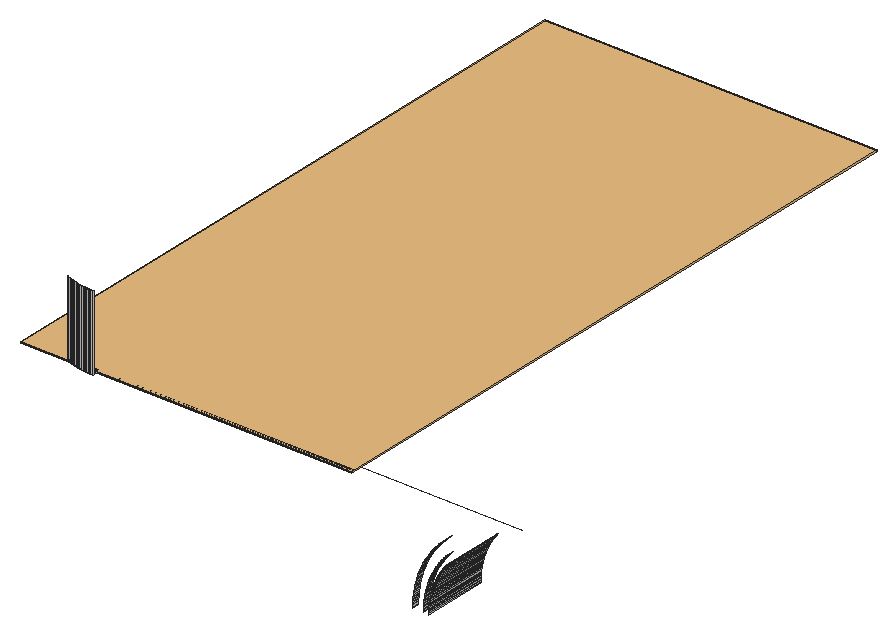
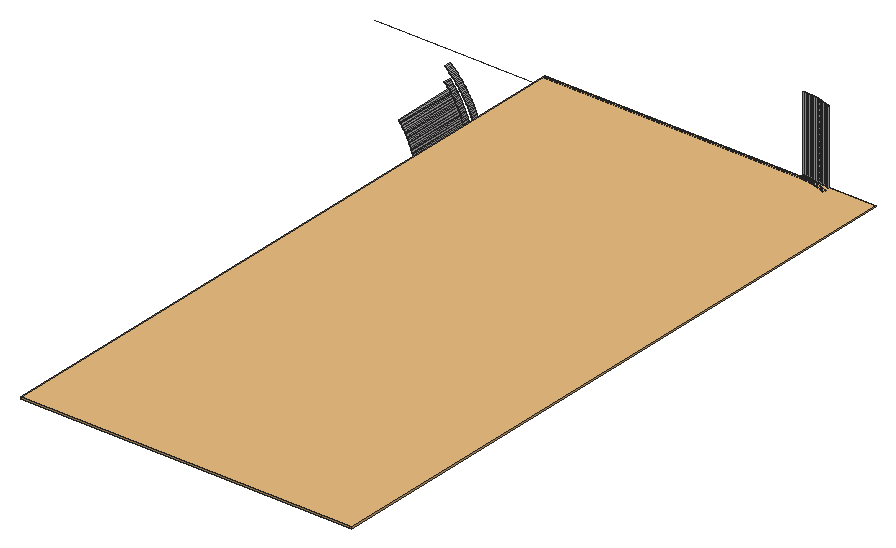
# SketchUp Ruby script. Lengths in inches.
U = 1.inch
M = Sketchup.active_model
def pt(a) = Geom::Point3d.new(a.map { |v| v * U })
def face(e, loops, mat)
  f = e.add_face(loops[0].map { |a| pt(a) })
  loops[1..].each { |l| e.add_face(l.map { |a| pt(a) }).erase! }
  f.material = f.back_material = mat if mat
  f
end
# faces: each face lists its corners as indices into pts; further lists are holes
def faces(e, pts, list, mat = nil) = list.each { |f| face(e, (f[0].is_a?(Array) ? f : [f]).map { |l| l.map { |i| pts[i] } }, mat) }
# xy, xz, yz: faces in a plane at the given z, y or x. An outline is a flat list of corners, or four numbers for a rectangle; further outlines are holes
def ring(l) = l.size == 4 ? [[l[0], l[1]], [l[2], l[1]], [l[2], l[3]], [l[0], l[3]]] : l.each_slice(2).to_a
def flat(e, list, mat, &to3) = list.each { |f| face(e, (f[0].is_a?(Array) ? f : [f]).map { |l| ring(l).map { |u, v| to3.(u, v) } }, mat) }
def xy(e, z, list, mat = nil) = flat(e, list, mat) { |x, y| [x, y, z] }
def xz(e, y, list, mat = nil) = flat(e, list, mat) { |x, z| [x, y, z] }
def yz(e, x, list, mat = nil) = flat(e, list, mat) { |y, z| [x, y, z] }
def lines(e, pts, list) = list.each { |a, b| e.add_line(pt(pts[a]), pt(pts[b])) }
# prism: a flat outline (further loops are holes) pulled along v
def prism(e, loops, v, mat = nil)
  f = face(e, loops, mat); d = Geom::Vector3d.new(v.map { |x| x * U })
  f.pushpull(f.normal.samedirection?(d) ? d.length : -d.length)
end
def box(e, o, s, mat = nil) = prism(e, [[o, [o[0] + s[0], o[1], o[2]], [o[0] + s[0], o[1] + s[1], o[2]], [o[0], o[1] + s[1], o[2]]]], [0, 0, s[2]], mat)
def at(x, y, z, deg = 0) = Geom::Transformation.translation(pt([x, y, z])) * Geom::Transformation.rotation(ORIGIN, Z_AXIS, deg.degrees)
def axes(o, x, y, z) = Geom::Transformation.new([*x, 0, *y, 0, *z, 0, *pt(o).to_a, 1])
def part(name) = M.definitions.add(name)
# library, detail: a bought-in or finely detailed component or shape, given as its bounding box
def library(name, o, s) = part(name).tap { |d| box(d.entities, o, s) }
def detail(e, o, s) = box(e.add_group.entities, o, s)
def put(e, d, t, mat = nil) = e.add_instance(d, t).tap { |i| i.material = mat if mat }
def group(e, t, mat = nil) = e.add_group.tap { |g| g.transformation = t; g.material = mat if mat }.entities
root = M.entities
M.materials.add("Outer Light - 1").color = [251, 216, 141]
M.materials.add("[Quartz Light Brown]").color = [215, 212, 212]
c1 = library("Group\#10",[0,0,0],[61.75,122.25,0.25])
xz(root,143,[[215.8,354,216,368]],"[Quartz Light Brown]")
xz(root,143.01,[[215.41,354,215.61,368]],"[Quartz Light Brown]")
xz(root,143.75,[[215.625,354,215.8125,354.25],[215.8125,354,216,354.25],[216,354,263.5,354.25]],"[Quartz Light Brown]")
xz(root,144.25,[[215.64,354,215.82,354.25],[215.82,354,216,354.25],[216,354,263.5,354.25]],"[Quartz Light Brown]")
yz(root,275.5,[[143,336,144.25,336.24]],"[Quartz Light Brown]")
yz(root,275.51,[[143,336.47,144.25,336.71]],"[Quartz Light Brown]")
yz(root,277.5,[[143,336,144.25,336.21]],"[Quartz Light Brown]")
yz(root,277.51,[[143,336.42,144.25,336.63]],"[Quartz Light Brown]")
yz(root,278.5,[[143,336,155,336.2]],"[Quartz Light Brown]")
yz(root,278.51,[[143,336.39,155,336.59]],"[Quartz Light Brown]")
p = [[275.51,144.25,336.47],[275.51,143,336.47],[275.5,143,336.24],[275.5,144.25,336.24],[277.5,143,336.21],[277.51,143,336.42],
  [277.51,144.25,336.42],[277.5,144.25,336.21],[278.51,143,336.39],[278.5,143,336.2],[278.5,155,336.2],[278.51,155,336.39],
  [277.51,143,336.63],[277.52,143,336.84],[277.52,144.25,336.84],[277.51,144.25,336.63],[278.52,143,336.79],[278.51,143,336.59],
  [278.51,155,336.59],[278.52,155,336.79],[275.52,144.25,336.94],[275.52,143,336.94],[275.51,143,336.71],[275.51,144.25,336.71],
  [277.53,143,337.05],[277.53,144.25,337.05],[278.53,143,336.98],[278.53,155,336.98],[275.54,144.25,337.18],[275.54,143,337.18],
  [277.55,143,337.26],[277.55,144.25,337.26],[278.55,143,337.18],[278.55,155,337.18],[275.56,144.25,337.41],[275.56,143,337.41],
  [278.5625,143,337.37],[278.5625,155,337.37],[277.57,143,337.46],[277.57,144.25,337.46],[275.58,144.25,337.65],[275.58,143,337.65],
  [278.58,143,337.57],[278.58,155,337.57],[277.59,143,337.67],[277.59,144.25,337.67],[275.6,144.25,337.88],[275.6,143,337.88],
  [278.6,143,337.76],[278.6,155,337.76],[277.61,143,337.88],[277.61,144.25,337.88],[278.63,143,337.96],[278.63,155,337.96],
  [275.625,144.25,338.12],[275.625,143,338.12],[277.64,143,338.09],[277.64,144.25,338.09],[278.66,143,338.15],[278.66,155,338.15],
  [275.65,144.25,338.35],[275.65,143,338.35],[277.67,143,338.3],[277.67,144.25,338.3],[278.68,143,338.35],[278.68,155,338.35],
  [275.6875,144.25,338.58],[275.6875,143,338.58],[277.7,143,338.5],[277.7,144.25,338.5],[278.72,143,338.54],[278.72,155,338.54],
  [277.73,143,338.71],[277.73,144.25,338.71],[278.75,143,338.73],[278.75,155,338.73],[275.72,144.25,338.82],[275.72,143,338.82],
  [277.77,143,338.92],[277.77,144.25,338.92],[278.79,143,338.93],[278.79,155,338.93],[275.76,144.25,339.05],[275.76,143,339.05],
  [277.81,143,339.12],[277.81,144.25,339.12],[278.83,143,339.12],[278.83,155,339.12],[275.8,144.25,339.28],[275.8,143,339.28],
  [277.85,143,339.33],[277.85,144.25,339.33],[278.87,143,339.31],[278.87,155,339.31],[275.85,144.25,339.51],[275.85,143,339.51],
  [277.89,143,339.53],[277.89,144.25,339.53],[278.91,143,339.5],[278.91,155,339.5],[275.89,144.25,339.74],[275.89,143,339.74],
  [277.94,143,339.74],[277.94,144.25,339.74],[278.96,143,339.69],[278.96,155,339.69],[275.94,144.25,339.97],[275.94,143,339.97],
  [277.99,143,339.9375],[277.99,144.25,339.9375],[279.01,143,339.88],[279.01,155,339.88],[278.05,143,340.14],[278.05,144.25,340.14],
  [279.0625,143,340.07],[279.0625,155,340.07],[276,144.25,340.2],[276,143,340.2],[278.1,143,340.34],[278.1,144.25,340.34],
  [279.12,143,340.26],[279.12,155,340.26],[276.05,144.25,340.43],[276.05,143,340.43],[278.16,143,340.54],[278.16,144.25,340.54],
  [279.17,143,340.45],[279.17,155,340.45],[276.11,144.25,340.66],[276.11,143,340.66],[279.23,143,340.64],[279.23,155,340.64],
  [278.22,143,340.74],[278.22,144.25,340.74],[279.3,143,340.82],[279.3,155,340.82],[276.18,144.25,340.89],[276.18,143,340.89],
  [278.28,143,340.94],[278.28,144.25,340.94],[279.36,143,341.01],[279.36,155,341.01],[276.24,144.25,341.11],[276.24,143,341.11],
  [278.35,143,341.14],[278.35,144.25,341.14],[279.43,143,341.19],[279.43,155,341.19],[276.31,144.25,341.34],[276.31,143,341.34],
  [278.42,143,341.34],[278.42,144.25,341.34],[279.5,143,341.375],[279.5,155,341.375],[276.38,144.25,341.5625],[276.38,143,341.5625],
  [278.49,143,341.54],[278.49,144.25,341.54],[279.57,143,341.56],[279.57,155,341.56],[278.5625,143,341.73],[278.5625,144.25,341.73],
  [276.46,144.25,341.79],[276.46,143,341.79],[279.64,143,341.74],[279.64,155,341.74],[278.64,143,341.93],[278.64,144.25,341.93],
  [279.72,143,341.92],[279.72,155,341.92],[276.53,144.25,342.01],[276.53,143,342.01],[278.72,143,342.12],[278.72,144.25,342.12],
  [279.8,143,342.1],[279.8,155,342.1],[276.61,144.25,342.23],[276.61,143,342.23],[278.8,143,342.32],[278.8,144.25,342.32],
  [279.88,143,342.28],[279.88,155,342.28],[276.7,144.25,342.45],[276.7,143,342.45],[278.88,143,342.51],[278.88,144.25,342.51],
  [279.96,143,342.46],[279.96,155,342.46],[276.78,144.25,342.67],[276.78,143,342.67],[278.97,143,342.7],[278.97,144.25,342.7],
  [280.05,143,342.63],[280.05,155,342.63],[280.13,143,342.81],[280.13,155,342.81],[276.87,144.25,342.89],[276.87,143,342.89],
  [279.06,143,342.89],[279.06,144.25,342.89],[280.23,143,342.98],[280.23,155,342.98],[276.96,144.25,343.11],[276.96,143,343.11],
  [279.15,143,343.08],[279.15,144.25,343.08],[280.32,143,343.16],[280.32,155,343.16],[277.06,144.25,343.32],[277.06,143,343.32],
  [279.24,143,343.26],[279.24,144.25,343.26],[280.41,143,343.33],[280.41,155,343.33],[277.15,144.25,343.54],[277.15,143,343.54],
  [279.34,143,343.45],[279.34,144.25,343.45],[280.51,143,343.5],[280.51,155,343.5],[279.4375,143,343.63],[279.4375,144.25,343.63],
  [277.25,144.25,343.75],[277.25,143,343.75],[280.61,143,343.67],[280.61,155,343.67],[279.54,143,343.82],[279.54,144.25,343.82],
  [277.36,144.25,343.96],[277.36,143,343.96],[280.71,143,343.84],[280.71,155,343.84],[279.64,143,344],[279.64,144.25,344],
  [280.8125,143,344],[280.8125,155,344],[277.46,144.25,344.17],[277.46,143,344.17],[279.75,143,344.18],[279.75,144.25,344.18],
  [280.92,143,344.17],[280.92,155,344.17],[277.57,144.25,344.38],[277.57,143,344.38],[279.86,143,344.36],[279.86,144.25,344.36],
  [281.03,143,344.33],[281.03,155,344.33],[281.14,143,344.5],[281.14,155,344.5],[277.68,144.25,344.59],[277.68,143,344.59],
  [279.97,143,344.54],[279.97,144.25,344.54],[280.08,143,344.71],[280.08,144.25,344.71],[281.25,143,344.66],[281.25,155,344.66],
  [277.8,144.25,344.8],[277.8,143,344.8],[280.2,143,344.89],[280.2,144.25,344.89],[281.36,143,344.82],[281.36,155,344.82],
  [277.91,144.25,345],[277.91,143,345],[281.48,143,344.97],[281.48,155,344.97],[280.3125,143,345.0625],[280.3125,144.25,345.0625],
  [278.03,144.25,345.2],[278.03,143,345.2],[281.6,143,345.13],[281.6,155,345.13],[280.43,143,345.23],[280.43,144.25,345.23],
  [281.72,143,345.29],[281.72,155,345.29],[278.15,144.25,345.4],[278.15,143,345.4],[280.56,143,345.4],[280.56,144.25,345.4],
  [281.84,143,345.44],[281.84,155,345.44],[278.28,144.25,345.61],[278.28,143,345.61],[280.68,143,345.57],[280.68,144.25,345.57],
  [278.4,144.25,345.8],[278.4,143,345.8],[280.81,143,345.74],[280.81,144.25,345.74],[280.93,143,345.91],[280.93,144.25,345.91],
  [278.53,144.25,346],[278.53,143,346],[281.07,143,346.07],[281.07,144.25,346.07],[278.67,144.25,346.2],[278.67,143,346.2],
  [281.2,143,346.23],[281.2,144.25,346.23],[278.8,144.25,346.39],[278.8,143,346.39],[281.33,143,346.39],[281.33,144.25,346.39],
  [278.9375,144.25,346.58],[278.9375,143,346.58],[281.47,143,346.55],[281.47,144.25,346.55],[281.61,143,346.71],[281.61,144.25,346.71],
  [279.08,144.25,346.77],[279.08,143,346.77],[281.75,143,346.86],[281.75,144.25,346.86],[279.22,144.25,346.96],[279.22,143,346.96],
  [281.89,143,347.01],[281.89,144.25,347.01],[279.36,144.25,347.14],[279.36,143,347.14],[279.51,144.25,347.33],[279.51,143,347.33],
  [279.66,144.25,347.51],[279.66,143,347.51],[279.8125,144.25,347.69],[279.8125,143,347.69],[279.97,144.25,347.87],[279.97,143,347.87],
  [280.125,144.25,348.04],[280.125,143,348.04],[280.28,144.25,348.22],[280.28,143,348.22],[280.44,144.25,348.39],[280.44,143,348.39],
  [280.61,144.25,348.56],[280.61,143,348.56],[280.77,144.25,348.73],[280.77,143,348.73],[280.94,144.25,348.89],[280.94,143,348.89],
  [281.11,144.25,349.06],[281.11,143,349.06],[281.28,144.25,349.22],[281.28,143,349.22],[281.46,144.25,349.375],[281.46,143,349.375],
  [281.63,144.25,349.53],[281.63,143,349.53],[281.81,144.25,349.6875],[281.81,143,349.6875],[214.63,143.0625,368],[214.63,143.0625,354],
  [214.82,143.05,354],[214.82,143.05,368],[215.02,143.03,354],[215.02,143.03,368],[215.21,143.02,354],[215.21,143.02,368],
  [215.41,143.01,354],[215.41,143.01,368],[215.61,143.01,368],[215.61,143.01,354],[215.8,143,354],[215.8,143,368],
  [213.85,143.16,368],[213.85,143.16,354],[214.04,143.13,354],[214.04,143.13,368],[214.24,143.1,354],[214.24,143.1,368],
  [214.43,143.08,354],[214.43,143.08,368],[213.27,143.25,368],[213.27,143.25,354],[213.46,143.22,354],[213.46,143.22,368],
  [213.65,143.18,354],[213.65,143.18,368],[212.69,143.37,368],[212.69,143.37,354],[212.88,143.33,354],[212.88,143.33,368],
  [213.07,143.29,354],[213.07,143.29,368],[212.31,143.46,368],[212.31,143.46,354],[212.5,143.41,354],[212.5,143.41,368],
  [211.93,143.5625,368],[211.93,143.5625,354],[212.12,143.51,354],[212.12,143.51,368],[211.55,143.67,368],[211.55,143.67,354],
  [211.74,143.62,354],[211.74,143.62,368],[211.18,143.8,368],[211.18,143.8,354],[211.36,143.73,354],[211.36,143.73,368],
  [210.99,143.86,368],[210.99,143.86,354],[214.33,143.85,354],[214.14,143.87,354],[214.14,143.87,354.25],[214.33,143.85,354.25],
  [214.51,143.83,354],[214.51,143.83,354.25],[214.7,143.81,354],[214.7,143.81,354.25],[214.88,143.79,354],[214.88,143.79,354.25],
  [215.07,143.78,354],[215.07,143.78,354.25],[215.25,143.77,354],[215.25,143.77,354.25],[215.44,143.76,354],[215.44,143.76,354.25],
  [215.625,143.75,354],[215.625,143.75,354.25],[210.625,144,368],[210.625,144,354],[210.81,143.93,354],[210.81,143.93,368],
  [213.77,143.93,354],[213.59,143.96,354],[213.59,143.96,354.25],[213.77,143.93,354.25],[213.96,143.9,354],[213.96,143.9,354.25],
  [210.44,144.07,368],[210.44,144.07,354],[213.22,144.02,354],[213.04,144.0625,354],[213.04,144.0625,354.25],[213.22,144.02,354.25],
  [213.4,143.99,354],[213.4,143.99,354.25],[210.26,144.14,368],[210.26,144.14,354],[212.67,144.14,354],[212.49,144.1875,354],
  [212.49,144.1875,354.25],[212.67,144.14,354.25],[212.86,144.1,354],[212.86,144.1,354.25],[212.3125,144.24,354],[212.13,144.29,354],
  [212.13,144.29,354.25],[212.3125,144.24,354.25],[211.95,144.34,354],[211.77,144.39,354],[211.77,144.39,354.25],[211.95,144.34,354.25],
  [214.21,144.37,354],[214.38,144.35,354],[214.38,144.35,354.25],[214.21,144.37,354.25],[214.5625,144.33,354],[214.5625,144.33,354.25],
  [214.74,144.31,354],[214.74,144.31,354.25],[214.92,144.29,354],[214.92,144.29,354.25],[215.1,144.28,354],[215.1,144.28,354.25],
  [215.28,144.27,354],[215.28,144.27,354.25],[215.46,144.26,354],[215.46,144.26,354.25],[215.64,144.25,354],[215.64,144.25,354.25],
  [211.6,144.45,354],[211.42,144.51,354],[211.42,144.51,354.25],[211.6,144.45,354.25],[213.49,144.48,354],[213.67,144.45,354],
  [213.67,144.45,354.25],[213.49,144.48,354.25],[213.85,144.42,354],[213.85,144.42,354.25],[214.03,144.39,354],[214.03,144.39,354.25],
  [211.24,144.57,354],[211.24,144.57,354.25],[213.14,144.55,354],[213.32,144.51,354],[213.32,144.51,354.25],[213.14,144.55,354.25],
  [211.07,144.63,354],[210.89,144.7,354],[210.89,144.7,354.25],[211.07,144.63,354.25],[212.62,144.67,354],[212.79,144.63,354],
  [212.79,144.63,354.25],[212.62,144.67,354.25],[212.97,144.59,354],[212.97,144.59,354.25],[210.72,144.76,354],[210.72,144.76,354.25],
  [212.27,144.77,354],[212.44,144.72,354],[212.44,144.72,354.25],[212.27,144.77,354.25],[210.55,144.83,354],[210.375,144.91,354],
  [210.375,144.91,354.25],[210.55,144.83,354.25],[211.92,144.87,354],[212.09,144.82,354],[212.09,144.82,354.25],[211.92,144.87,354.25],
  [210.2,144.98,354],[210.2,144.98,354.25],[211.58,144.98,354],[211.75,144.92,354],[211.75,144.92,354.25],[211.58,144.98,354.25],
  [211.24,145.1,354],[211.41,145.04,354],[211.41,145.04,354.25],[211.24,145.1,354.25],[211.07,145.16,354],[211.07,145.16,354.25],
  [210.74,145.3,354],[210.9,145.23,354],[210.9,145.23,354.25],[210.74,145.3,354.25],[210.57,145.37,354],[210.57,145.37,354.25],
  [210.24,145.51,354],[210.41,145.4375,354],[210.41,145.4375,354.25],[210.24,145.51,354.25],[263.5,146,354],[293.5,146,354]]
faces(root,p,[[0,1,2,3],[4,5,6,7],[8,9,10,11],[12,13,14,15],[16,17,18,19],[20,21,22,23],[13,24,25,14],[26,16,19,27],
  [28,29,21,20],[24,30,31,25],[32,26,27,33],[34,35,29,28],[36,32,33,37],[30,38,39,31],[40,41,35,34],[42,36,37,43],
  [38,44,45,39],[46,47,41,40],[48,42,43,49],[44,50,51,45],[52,48,49,53],[54,55,47,46],[50,56,57,51],[58,52,53,59],
  [60,61,55,54],[56,62,63,57],[64,58,59,65],[66,67,61,60],[62,68,69,63],[70,64,65,71],[68,72,73,69],[74,70,71,75],
  [76,77,67,66],[72,78,79,73],[80,74,75,81],[82,83,77,76],[78,84,85,79],[86,80,81,87],[88,89,83,82],[84,90,91,85],
  [92,86,87,93],[94,95,89,88],[90,96,97,91],[98,92,93,99],[100,101,95,94],[96,102,103,97],[104,98,99,105],[106,107,101,100],
  [102,108,109,103],[110,104,105,111],[108,112,113,109],[114,110,111,115],[116,117,107,106],[112,118,119,113],[120,114,115,121],[122,123,117,116],
  [118,124,125,119],[126,120,121,127],[128,129,123,122],[130,126,127,131],[124,132,133,125],[134,130,131,135],[136,137,129,128],[132,138,139,133],
  [140,134,135,141],[142,143,137,136],[138,144,145,139],[146,140,141,147],[148,149,143,142],[144,150,151,145],[152,146,147,153],[154,155,149,148],
  [150,156,157,151],[158,152,153,159],[156,160,161,157],[162,163,155,154],[164,158,159,165],[160,166,167,161],[168,164,165,169],[170,171,163,162],
  [166,172,173,167],[174,168,169,175],[176,177,171,170],[172,178,179,173],[180,174,175,181],[182,183,177,176],[178,184,185,179],[186,180,181,187],
  [188,189,183,182],[184,190,191,185],[192,186,187,193],[194,192,193,195],[196,197,189,188],[190,198,199,191],[200,194,195,201],[202,203,197,196],
  [198,204,205,199],[206,200,201,207],[208,209,203,202],[204,210,211,205],[212,206,207,213],[214,215,209,208],[210,216,217,211],[218,212,213,219],
  [216,220,221,217],[222,223,215,214],[224,218,219,225],[220,226,227,221],[228,229,223,222],[230,224,225,231],[226,232,233,227],[234,230,231,235],
  [236,237,229,228],[232,238,239,233],[240,234,235,241],[242,243,237,236],[238,244,245,239],[246,240,241,247],[248,246,247,249],[250,251,243,242],
  [244,252,253,245],[252,254,255,253],[256,248,249,257],[258,259,251,250],[254,260,261,255],[262,256,257,263],[264,265,259,258],[266,262,263,267],
  [260,268,269,261],[270,271,265,264],[272,266,267,273],[268,274,275,269],[276,272,273,277],[278,279,271,270],[274,280,281,275],[282,276,277,283],
  [284,285,279,278],[280,286,287,281],[288,289,285,284],[286,290,291,287],[290,292,293,291],[294,295,289,288],[292,296,297,293],[298,299,295,294],
  [296,300,301,297],[302,303,299,298],[300,304,305,301],[306,307,303,302],[304,308,309,305],[308,310,311,309],[312,313,307,306],[310,314,315,311],
  [316,317,313,312],[314,318,319,315],[320,321,317,316],[322,323,321,320],[324,325,323,322],[326,327,325,324],[328,329,327,326],[330,331,329,328],
  [332,333,331,330],[334,335,333,332],[336,337,335,334],[338,339,337,336],[340,341,339,338],[342,343,341,340],[344,345,343,342],[346,347,345,344],
  [348,349,347,346],[350,351,349,348],[352,353,354,355],[355,354,356,357],[357,356,358,359],[359,358,360,361],[362,363,364,365],[366,367,368,369],
  [369,368,370,371],[371,370,372,373],[373,372,353,352],[374,375,376,377],[377,376,378,379],[379,378,367,366],[380,381,382,383],[383,382,384,385],
  [385,384,375,374],[386,387,388,389],[389,388,381,380],[390,391,392,393],[393,392,387,386],[394,395,396,397],[397,396,391,390],[398,399,400,401],
  [401,400,395,394],[402,403,399,398],[404,405,406,407],[408,404,407,409],[410,408,409,411],[412,410,411,413],[414,412,413,415],[416,414,415,417],
  [418,416,417,419],[420,418,419,421],[422,423,424,425],[425,424,403,402],[426,427,428,429],[430,426,429,431],[405,430,431,406],[432,433,423,422],
  [434,435,436,437],[438,434,437,439],[427,438,439,428],[440,441,433,432],[442,443,444,445],[446,442,445,447],[435,446,447,436],[448,449,450,451],
  [443,448,451,444],[452,453,454,455],[449,452,455,450],[456,457,458,459],[457,460,461,458],[460,462,463,461],[462,464,465,463],[464,466,467,465],
  [466,468,469,467],[468,470,471,469],[470,472,473,471],[474,475,476,477],[453,474,477,454],[478,479,480,481],[479,482,483,480],[482,484,485,483],
  [484,456,459,485],[475,486,487,476],[488,489,490,491],[489,478,481,490],[492,493,494,495],[486,492,495,487],[496,497,498,499],[497,500,501,498],
  [500,488,491,501],[493,502,503,494],[504,505,506,507],[505,496,499,506],[508,509,510,511],[502,508,511,503],[512,513,514,515],[513,504,507,514],
  [509,516,517,510],[518,519,520,521],[519,512,515,520],[522,523,524,525],[523,518,521,524],[526,522,525,527],[528,529,530,531],[529,526,527,530],
  [532,528,531,533],[534,535,536,537],[535,532,533,536]],"[Quartz Light Brown]")
lines(root,p,[[538,539]])
put(root,c1,at(201.75,143.75,354),"Outer Light - 1")
